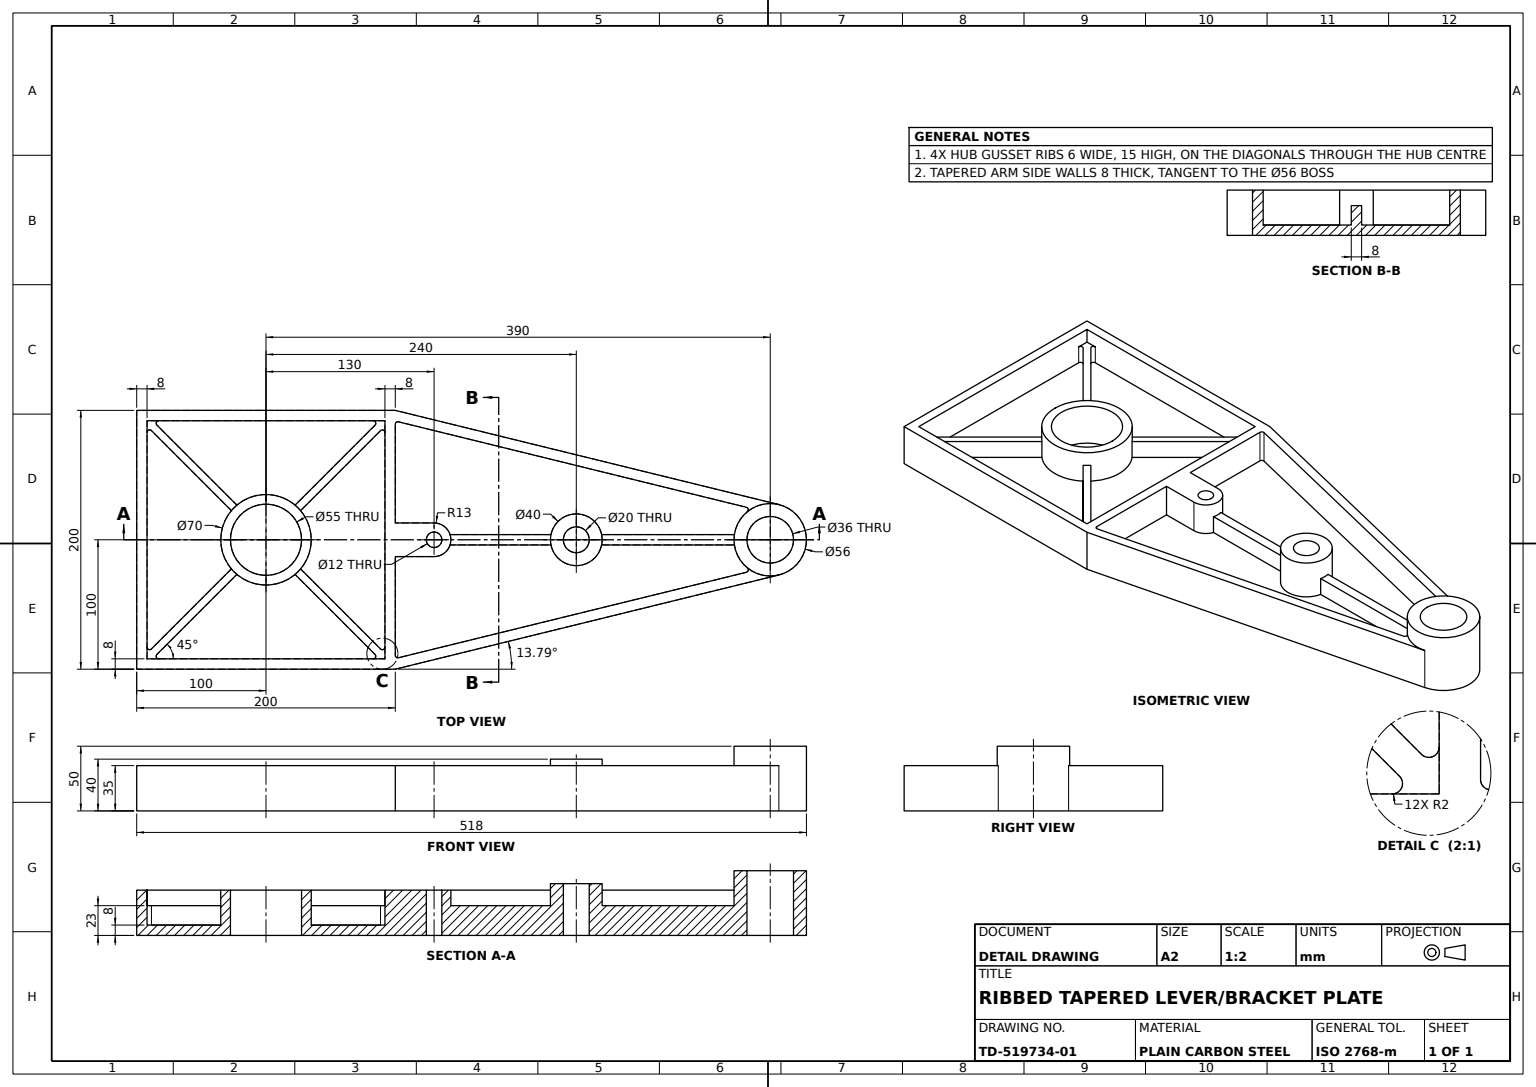
solid
v1 (92,8,-92)
v2 (91.816521,8,-92)
e1 v1 v2 LINE
v3 (92,35,-92)
e2 v3 v1 LINE
v4 (-92,35,-92)
e3 v3 v4 LINE
v5 (-92,8,-92)
e4 v4 v5 LINE
v6 (-91.816521,8,-92)
e5 v6 v5 LINE
v7 (-91.816521,23,-92)
e6 v6 v7 LINE
v8 (-82.913661,23,-92)
e7 v8 v7 LINE
v9 (-82.913661,8,-92)
e8 v8 v9 LINE
v10 (82.944203,8,-92)
e9 v10 v9 LINE
v11 (82.944203,23,-92)
e10 v10 v11 LINE
v12 (91.816521,23,-92)
e11 v12 v11 LINE
e12 v12 v2 LINE
face PLANE(AX(P(-92,35,-92),D(0,0,1),D(1,0,0))) [-e1 -e2 e3 e4 -e5 e6 -e7 e8 -e9 e10 -e11 e12]
v13 (-4,23,-220.404082)
v14 (-4,23,-142.369317)
e13 v13 v14 LINE
v15 (0,23,-143)
e14 v14 v15 CIRCLE(AX(P(0,23,-130),D(0,-1,0),D(0,0,-1)),13)
v16 (4,23,-142.369317)
e15 v15 v16 CIRCLE(AX(P(0,23,-130),D(0,-1,0),D(0,0,-1)),13)
v17 (4,23,-220.404082)
e16 v16 v17 LINE
v18 (0,23,-220)
e17 v17 v18 CIRCLE(AX(P(0,23,-240),D(0,-1,0),D(0,0,-1)),20)
e18 v18 v13 CIRCLE(AX(P(0,23,-240),D(0,-1,0),D(0,0,-1)),20)
face PLANE(AX(P(0,23,0),D(0,-1,0),D(0,0,-1))) rev [e13 e14 e15 e16 e17 e18]
v19 (-22.544627,23,26.771996)
v20 (-22.544627,8,26.771996)
e19 v19 v20 LINE
v21 (-84.358417,23,88.585786)
e20 v21 v19 LINE
v22 (-84.358417,8,88.585786)
e21 v21 v22 LINE
e22 v22 v20 LINE
face PLANE(AX(P(-89.794576,23,94.021945),D(-0.707106781,0,-0.707106781),D(-0.707106781,0,0.707106781))) rev [-e19 -e20 e21 e22]
v23 (92,23,91.816521)
v24 (92,8,91.816521)
e23 v23 v24 LINE
v25 (91.816521,23,92)
e24 v25 v23 LINE
v26 (91.816521,8,92)
e25 v26 v25 LINE
e26 v26 v24 LINE
face PLANE(AX(P(94.021945,23,89.794576),D(-0.707106781,0,-0.707106781),D(-0.707106781,0,0.707106781))) rev [-e23 -e24 -e25 e26]
v27 (25.14377,35,-371.458403)
v28 (25.14377,8,-371.458403)
e27 v27 v28 LINE
v29 (23.201406,35,-372.981725)
e28 v29 v27 CIRCLE(AX(P(23.201406,35,-370.981725),D(0,-1,0),D(0,0,1)),2)
v30 (23.201406,8,-372.981725)
e29 v29 v30 LINE
e30 v28 v30 CIRCLE(AX(P(23.201406,8,-370.981725),D(0,1,0),D(0,0,1)),2)
face CYL(AX(P(23.201406,8,-370.981725),D(0,-1,0),D(0,0,-1)),2) rev [-e27 -e28 e29 -e30]
v31 (-89.212448,35,-100)
v32 (-91.154812,35,-102.476677)
e31 v31 v32 CIRCLE(AX(P(-89.212448,35,-102),D(0,-1,0),D(0,0,1)),2)
v33 (-25.14377,35,-371.458403)
e32 v33 v32 LINE
v34 (-23.201406,35,-372.981725)
e33 v33 v34 CIRCLE(AX(P(-23.201406,35,-370.981725),D(0,-1,0),D(0,0,1)),2)
v35 (-21.654645,35,-372.24961)
e34 v34 v35 CIRCLE(AX(P(-23.201406,35,-370.981725),D(0,-1,0),D(0,0,1)),2)
v36 (-27.193099,35,-396.673482)
e35 v35 v36 CIRCLE(AX(P(0,35,-390),D(0,-1,0),D(0,0,1)),28)
v37 (-100,35,-100)
e36 v36 v37 LINE
v38 (-100,35,100)
e37 v37 v38 LINE
v39 (100,35,100)
e38 v38 v39 LINE
v40 (100,35,-100)
e39 v39 v40 LINE
v41 (27.193099,35,-396.673482)
e40 v40 v41 LINE
v42 (21.654645,35,-372.24961)
e41 v41 v42 CIRCLE(AX(P(0,35,-390),D(0,-1,0),D(0,0,1)),28)
e42 v42 v29 CIRCLE(AX(P(23.201406,35,-370.981725),D(0,-1,0),D(0,0,1)),2)
v43 (91.154812,35,-102.476677)
e43 v43 v27 LINE
v44 (89.212448,35,-100)
e44 v43 v44 CIRCLE(AX(P(89.212448,35,-102),D(0,-1,0),D(0,0,1)),2)
v45 (13,35,-100)
e45 v44 v45 LINE
v46 (13,35,-130)
e46 v45 v46 LINE
v47 (0,35,-143)
e47 v46 v47 CIRCLE(AX(P(0,35,-130),D(0,1,0),D(0,0,1)),13)
v48 (-13,35,-130)
e48 v47 v48 CIRCLE(AX(P(0,35,-130),D(0,1,0),D(0,0,1)),13)
v49 (-13,35,-100)
e49 v48 v49 LINE
e50 v49 v31 LINE
v50 (0,35,-136)
v51 (0,35,-124)
e51 v50 v51 CIRCLE(AX(P(0,35,-130),D(0,1,0),D(0,0,1)),6)
e52 v51 v50 CIRCLE(AX(P(0,35,-130),D(0,1,0),D(0,0,1)),6)
v52 (92,35,92)
e53 v52 v3 LINE
v53 (-92,35,92)
e54 v53 v52 LINE
e55 v4 v53 LINE
face PLANE(AX(P(0,35,0),D(0,1,0),D(0,0,1))) [e31 -e32 e33 e34 e35 e36 e37 e38 e39 e40 e41 e42 e28 -e43 e44 e45 e46 e47 e48 e49 e50] [-e51 -e52] [-e53 -e54 -e55 -e3]
v54 (-26.785954,23,22.528042)
v55 (-88.585786,23,84.327874)
e56 v54 v55 LINE
v56 (-26.785954,8,22.528042)
e57 v54 v56 LINE
v57 (-88.585786,8,84.327874)
e58 v56 v57 LINE
e59 v57 v55 LINE
face PLANE(AX(P(-94.037217,23,89.779305),D(0.707106781,0,0.707106781),D(0.707106781,0,-0.707106781))) rev [-e56 e57 e58 e59]
v58 (-21.654645,8,-372.24961)
v59 (-23.201406,8,-372.981725)
e60 v58 v59 CIRCLE(AX(P(-23.201406,8,-370.981725),D(0,1,0),D(0,0,1)),2)
e61 v35 v58 LINE
e62 v34 v59 LINE
face CYL(AX(P(-23.201406,8,-370.981725),D(0,-1,0),D(0,0,-1)),2) rev [-e60 -e61 -e34 e62]
v60 (0,50,-372)
v61 (0,0,-372)
e63 v60 v61 LINE
v62 (0,0,-408)
e64 v61 v62 CIRCLE(AX(P(0,0,-390),D(0,-1,0),D(0,0,-1)),18)
v63 (0,50,-408)
e65 v63 v62 LINE
e66 v60 v63 CIRCLE(AX(P(0,50,-390),D(0,-1,0),D(0,0,-1)),18)
face CYL(AX(P(0,50,-390),D(0,-1,0),D(0,0,-1)),18) rev [e63 e64 -e65 -e66]
v64 (-4,23,-362.287187)
v65 (-4,23,-259.595918)
e67 v64 v65 LINE
v66 (-4,8,-362.287187)
e68 v64 v66 LINE
v67 (-4,8,-259.595918)
e69 v66 v67 LINE
e70 v67 v65 LINE
face PLANE(AX(P(-4,23,-100.849632),D(1,0,0),D(0,0,-1))) rev [-e67 e68 e69 e70]
v68 (-13,8,-130)
v69 (-13,8,-100)
e71 v68 v69 LINE
e72 v49 v69 LINE
e73 v48 v68 LINE
face PLANE(AX(P(-13,85.249378,-130),D(1,0,0),D(0,0,-1))) rev [e71 -e72 -e49 e73]
e74 v47 v15 LINE
v70 (-4,8,-142.369317)
e75 v70 v14 LINE
e76 v70 v68 CIRCLE(AX(P(0,8,-130),D(0,1,0),D(0,0,1)),13)
face CYL(AX(P(0,85.249378,-130),D(0,-1,0),D(0,0,-1)),13) [-e48 e74 -e14 -e75 e76 -e73]
v71 (13,8,-130)
v72 (4,8,-142.369317)
e77 v71 v72 CIRCLE(AX(P(0,8,-130),D(0,1,0),D(0,0,1)),13)
e78 v16 v72 LINE
e79 v46 v71 LINE
face CYL(AX(P(0,85.249378,-130),D(0,-1,0),D(0,0,-1)),13) [e77 -e78 -e15 -e74 -e47 e79]
v73 (-89.212448,8,-100)
e80 v69 v73 LINE
e81 v73 v31 LINE
face PLANE(AX(P(-100,35,-100),D(0,0,1),D(1,0,0))) rev [e72 e80 e81 -e50]
v74 (-92,23,-91.816521)
v75 (-92,8,-91.816521)
e82 v74 v75 LINE
e83 v7 v74 LINE
e84 v6 v75 LINE
face PLANE(AX(P(-94.021945,23,-89.794576),D(0.707106781,0,0.707106781),D(0.707106781,0,-0.707106781))) rev [-e82 -e83 -e6 e84]
v76 (92,23,82.944203)
v77 (90,23,84.944203)
e85 v76 v77 CIRCLE(AX(P(90,23,82.944203),D(0,-1,0),D(0,0,1)),2)
v78 (88.585786,23,84.358417)
e86 v77 v78 CIRCLE(AX(P(90,23,82.944203),D(0,-1,0),D(0,0,1)),2)
v79 (26.771996,23,22.544627)
e87 v78 v79 LINE
v80 (22.528042,23,26.785954)
e88 v80 v79 CIRCLE(AX(P(0,23,0),D(0,1,0),D(0,0,1)),35)
v81 (84.327874,23,88.585786)
e89 v80 v81 LINE
v82 (82.913661,23,92)
e90 v81 v82 CIRCLE(AX(P(82.913661,23,90),D(0,-1,0),D(0,0,1)),2)
e91 v82 v25 LINE
e92 v23 v76 LINE
face PLANE(AX(P(0,23,0),D(0,1,0),D(0,0,1))) [e85 e86 e87 -e88 e89 e90 e91 e24 e92]
v83 (-88.585786,8,-84.358417)
v84 (-92,8,-82.944203)
e93 v83 v84 CIRCLE(AX(P(-90,8,-82.944203),D(0,1,0),D(0,0,1)),2)
v85 (-88.585786,23,-84.358417)
e94 v85 v83 LINE
v86 (-92,23,-82.944203)
e95 v86 v85 CIRCLE(AX(P(-90,23,-82.944203),D(0,-1,0),D(0,0,1)),2)
e96 v84 v86 LINE
face CYL(AX(P(-90,35,-82.944203),D(0,1,0),D(0,0,1)),2) rev [-e93 -e94 -e95 -e96]
v87 (21.654645,8,-372.24961)
e97 v30 v87 CIRCLE(AX(P(23.201406,8,-370.981725),D(0,1,0),D(0,0,1)),2)
e98 v87 v42 LINE
face CYL(AX(P(23.201406,8,-370.981725),D(0,-1,0),D(0,0,-1)),2) rev [-e97 -e29 -e42 -e98]
v88 (-92,8,91.816521)
v89 (-92,23,91.816521)
e99 v88 v89 LINE
v90 (-91.816521,8,92)
e100 v88 v90 LINE
v91 (-91.816521,23,92)
e101 v91 v90 LINE
e102 v89 v91 LINE
face PLANE(AX(P(-89.794576,23,94.021945),D(0.707106781,0,-0.707106781),D(-0.707106781,0,-0.707106781))) rev [-e99 e100 -e101 -e102]
v92 (-25.14377,8,-371.458403)
e103 v92 v33 LINE
e104 v59 v92 CIRCLE(AX(P(-23.201406,8,-370.981725),D(0,1,0),D(0,0,1)),2)
face CYL(AX(P(-23.201406,8,-370.981725),D(0,-1,0),D(0,0,-1)),2) rev [-e33 -e103 -e104 -e62]
v93 (82.913661,8,92)
v94 (84.327874,8,88.585786)
e105 v93 v94 CIRCLE(AX(P(82.913661,8,90),D(0,1,0),D(0,0,1)),2)
e106 v82 v93 LINE
e107 v94 v81 LINE
face CYL(AX(P(82.913661,35,90),D(0,-1,0),D(0,0,-1)),2) rev [-e105 -e106 -e90 -e107]
v95 (-4,8,-220.404082)
e108 v95 v70 LINE
e109 v13 v95 LINE
face PLANE(AX(P(-4,23,-100.849632),D(1,0,0),D(0,0,-1))) rev [e108 e75 -e13 e109]
v96 (-100,0,100)
e110 v38 v96 LINE
v97 (100,0,100)
e111 v96 v97 LINE
e112 v39 v97 LINE
face PLANE(AX(P(-100,8,100),D(0,0,-1),D(-1,0,0))) rev [-e38 e110 e111 -e112]
v98 (-82.944203,23,92)
e113 v98 v21 CIRCLE(AX(P(-82.944203,23,90),D(0,-1,0),D(0,0,1)),2)
e114 v54 v19 CIRCLE(AX(P(0,23,0),D(0,1,0),D(0,0,1)),35)
v99 (-92,23,82.913661)
e115 v55 v99 CIRCLE(AX(P(-90,23,82.913661),D(0,-1,0),D(0,0,1)),2)
e116 v99 v89 LINE
e117 v91 v98 LINE
face PLANE(AX(P(0,23,0),D(0,1,0),D(0,0,1))) [e113 e20 -e114 e56 e115 e116 e102 e117]
v100 (-91.154812,8,-102.476677)
e118 v32 v100 LINE
e119 v92 v100 LINE
face PLANE(AX(P(-89.799329,417.460455,-108),D(0.971182107,0,0.238338657),D(0.238338657,0,-0.971182107))) [e103 e32 e118 -e119]
e120 v74 v86 LINE
e121 v5 v75 LINE
v101 (-92,8,92)
e122 v53 v101 LINE
e123 v88 v101 LINE
v102 (-92,8,82.913661)
e124 v99 v102 LINE
e125 v84 v102 LINE
face PLANE(AX(P(-92,35,92),D(1,0,0),D(0,0,-1))) [e96 -e120 e82 -e121 -e4 e55 e122 -e123 e99 -e116 e124 -e125]
v103 (0,40,-230)
v104 (0,0,-230)
e126 v103 v104 LINE
v105 (0,0,-250)
e127 v104 v105 CIRCLE(AX(P(0,0,-240),D(0,-1,0),D(0,0,-1)),10)
v106 (0,40,-250)
e128 v106 v105 LINE
e129 v106 v103 CIRCLE(AX(P(0,40,-240),D(0,1,0),D(0,0,1)),10)
face CYL(AX(P(0,50,-240),D(0,-1,0),D(0,0,-1)),10) rev [e126 e127 -e128 e129]
v107 (-84.327874,8,-88.585786)
e130 v9 v107 CIRCLE(AX(P(-82.913661,8,-90),D(0,1,0),D(0,0,1)),2)
v108 (-22.528042,8,-26.785954)
e131 v108 v107 LINE
v109 (0,8,-35)
e132 v109 v108 CIRCLE(AX(P(0,8,0),D(0,1,0),D(0,0,1)),35)
v110 (22.544627,8,-26.771996)
e133 v110 v109 CIRCLE(AX(P(0,8,0),D(0,1,0),D(0,0,1)),35)
v111 (84.358417,8,-88.585786)
e134 v111 v110 LINE
e135 v111 v10 CIRCLE(AX(P(82.944203,8,-90),D(0,1,0),D(0,0,1)),2)
face PLANE(AX(P(0,8,-390),D(0,1,0),D(0,0,1))) [e130 -e131 -e132 -e133 -e134 e135 e9]
v112 (-84.327874,23,-88.585786)
e136 v107 v112 LINE
e137 v112 v8 CIRCLE(AX(P(-82.913661,23,-90),D(0,-1,0),D(0,0,1)),2)
face CYL(AX(P(-82.913661,35,-90),D(0,-1,0),D(0,0,-1)),2) rev [-e136 -e130 -e8 -e137]
v113 (88.585786,8,84.358417)
e138 v78 v113 LINE
v114 (90,8,84.944203)
e139 v114 v77 LINE
e140 v113 v114 CIRCLE(AX(P(90,8,82.944203),D(0,1,0),D(0,0,1)),2)
face CYL(AX(P(90,35,82.944203),D(0,1,0),D(0,0,1)),2) rev [-e138 -e86 -e139 -e140]
v115 (0,0,-136)
e141 v50 v115 LINE
v116 (0,0,-124)
e142 v115 v116 CIRCLE(AX(P(0,0,-130),D(0,-1,0),D(0,0,-1)),6)
e143 v51 v116 LINE
face CYL(AX(P(0,50,-130),D(0,-1,0),D(0,0,-1)),6) rev [e52 e141 e142 -e143]
v117 (-82.944203,8,92)
e144 v22 v117 CIRCLE(AX(P(-82.944203,8,90),D(0,1,0),D(0,0,1)),2)
e145 v117 v93 LINE
v118 (22.528042,8,26.785954)
e146 v118 v94 LINE
v119 (0,8,35)
e147 v119 v118 CIRCLE(AX(P(0,8,0),D(0,1,0),D(0,0,1)),35)
e148 v20 v119 CIRCLE(AX(P(0,8,0),D(0,1,0),D(0,0,1)),35)
face PLANE(AX(P(0,8,-390),D(0,1,0),D(0,0,1))) [e144 e145 e105 -e146 -e147 -e148 -e22]
v120 (0,23,-260)
e149 v65 v120 CIRCLE(AX(P(0,23,-240),D(0,-1,0),D(0,0,-1)),20)
v121 (4,23,-259.595918)
e150 v120 v121 CIRCLE(AX(P(0,23,-240),D(0,-1,0),D(0,0,-1)),20)
v122 (4,23,-362.287187)
e151 v121 v122 LINE
v123 (0,23,-362)
e152 v122 v123 CIRCLE(AX(P(0,23,-390),D(0,-1,0),D(0,0,-1)),28)
e153 v123 v64 CIRCLE(AX(P(0,23,-390),D(0,-1,0),D(0,0,-1)),28)
face PLANE(AX(P(0,23,0),D(0,-1,0),D(0,0,-1))) rev [e67 e149 e150 e151 e152 e153]
v124 (-26.771996,23,-22.544627)
e154 v85 v124 LINE
v125 (-22.528042,23,-26.785954)
e155 v125 v124 CIRCLE(AX(P(0,23,0),D(0,1,0),D(0,0,1)),35)
e156 v125 v112 LINE
face PLANE(AX(P(0,23,0),D(0,1,0),D(0,0,1))) [e7 e83 e120 e95 e154 -e155 e156 e137]
v126 (26.771996,8,22.544627)
e157 v113 v126 LINE
v127 (92,8,82.944203)
e158 v114 v127 CIRCLE(AX(P(90,8,82.944203),D(0,1,0),D(0,0,1)),2)
v128 (92,8,-82.913661)
e159 v127 v128 LINE
v129 (90,8,-84.913661)
e160 v128 v129 CIRCLE(AX(P(90,8,-82.913661),D(0,1,0),D(0,0,1)),2)
v130 (88.585786,8,-84.327874)
e161 v129 v130 CIRCLE(AX(P(90,8,-82.913661),D(0,1,0),D(0,0,1)),2)
v131 (26.785954,8,-22.528042)
e162 v131 v130 LINE
e163 v126 v131 CIRCLE(AX(P(0,8,0),D(0,1,0),D(0,0,1)),35)
face PLANE(AX(P(0,8,-390),D(0,1,0),D(0,0,1))) [-e157 e140 e158 e159 e160 e161 -e162 -e163]
v132 (84.358417,23,-88.585786)
e164 v11 v132 CIRCLE(AX(P(82.944203,23,-90),D(0,-1,0),D(0,0,1)),2)
e165 v132 v111 LINE
face CYL(AX(P(82.944203,35,-90),D(0,1,0),D(0,0,1)),2) rev [-e164 -e10 -e135 -e165]
e166 v103 v106 CIRCLE(AX(P(0,40,-240),D(0,1,0),D(0,0,1)),10)
e167 v105 v104 CIRCLE(AX(P(0,0,-240),D(0,-1,0),D(0,0,-1)),10)
face CYL(AX(P(0,50,-240),D(0,-1,0),D(0,0,-1)),10) rev [e166 e128 e167 -e126]
v133 (0,50,-362)
e168 v133 v123 LINE
v134 (0,50,-418)
e169 v134 v133 CIRCLE(AX(P(0,50,-390),D(0,1,0),D(0,0,1)),28)
v135 (0,0,-418)
e170 v134 v135 LINE
v136 (-27.193099,0,-396.673482)
e171 v135 v136 CIRCLE(AX(P(0,0,-390),D(0,1,0),D(0,0,1)),28)
e172 v36 v136 LINE
e173 v58 v66 CIRCLE(AX(P(0,8,-390),D(0,1,0),D(0,0,1)),28)
face CYL(AX(P(0,8,-390),D(0,-1,0),D(0,0,-1)),28) [-e153 -e168 -e169 e170 e171 -e172 -e35 e61 e173 -e68]
e174 v127 v76 LINE
face CYL(AX(P(90,35,82.944203),D(0,1,0),D(0,0,1)),2) rev [-e158 e139 -e85 -e174]
v137 (22.544627,23,-26.771996)
e175 v137 v110 LINE
v138 (0,35,-35)
e176 v138 v109 LINE
v139 (0,35,35)
e177 v139 v138 CIRCLE(AX(P(0,35,0),D(0,1,0),D(0,0,1)),35)
e178 v139 v119 LINE
e179 v80 v118 LINE
e180 v79 v126 LINE
v140 (26.785954,23,-22.528042)
e181 v140 v131 LINE
e182 v140 v137 CIRCLE(AX(P(0,23,0),D(0,1,0),D(0,0,1)),35)
face CYL(AX(P(0,35,0),D(0,-1,0),D(0,0,-1)),35) [e175 e133 -e176 -e177 e178 e147 -e179 e88 e180 e163 -e181 e182]
v141 (92,8,-91.816521)
e183 v141 v1 LINE
e184 v141 v2 LINE
face PLANE(AX(P(0,8,-390),D(0,1,0),D(0,0,1))) [e183 e1 -e184]
v142 (92,8,92)
e185 v26 v142 LINE
e186 v142 v24 LINE
face PLANE(AX(P(0,8,-390),D(0,1,0),D(0,0,1))) [e185 e186 -e26]
e187 v116 v115 CIRCLE(AX(P(0,0,-130),D(0,-1,0),D(0,0,-1)),6)
face CYL(AX(P(0,50,-130),D(0,-1,0),D(0,0,-1)),6) rev [-e141 e51 e143 e187]
v143 (0,0,27.5)
v144 (0,0,-27.5)
e188 v143 v144 CIRCLE(AX(P(0,0,0),D(0,-1,0),D(0,0,-1)),27.5)
v145 (0,35,-27.5)
e189 v145 v144 LINE
v146 (0,35,27.5)
e190 v145 v146 CIRCLE(AX(P(0,35,0),D(0,1,0),D(0,0,1)),27.5)
e191 v146 v143 LINE
face CYL(AX(P(0,50,0),D(0,-1,0),D(0,0,-1)),27.5) rev [e188 -e189 e190 e191]
v147 (-100,0,-100)
e192 v37 v147 LINE
e193 v147 v96 LINE
face PLANE(AX(P(-100,8,100),D(1,0,0),D(0,0,-1))) rev [-e110 -e37 e192 e193]
face PLANE(AX(P(94.021945,23,89.794576),D(-0.707106781,0,0.707106781),D(0.707106781,0,0.707106781))) rev [e138 e157 -e180 -e87]
e194 v144 v143 CIRCLE(AX(P(0,0,0),D(0,-1,0),D(0,0,-1)),27.5)
e195 v146 v145 CIRCLE(AX(P(0,35,0),D(0,1,0),D(0,0,1)),27.5)
face CYL(AX(P(0,50,0),D(0,-1,0),D(0,0,-1)),27.5) rev [e194 -e191 e195 e189]
v148 (100,0,-100)
e196 v97 v148 LINE
e197 v40 v148 LINE
face PLANE(AX(P(100,8,100),D(-1,0,0),D(0,0,1))) rev [-e39 e112 e196 -e197]
v149 (91.154812,8,-102.476677)
e198 v149 v28 LINE
e199 v149 v43 LINE
face PLANE(AX(P(19.423642,417.460455,-394.766773),D(-0.971182107,0,0.238338657),D(0.238338657,0,0.971182107))) [e27 -e198 e199 e43]
v150 (13,8,-100)
e200 v45 v150 LINE
e201 v150 v71 LINE
face PLANE(AX(P(13,85.249378,-130),D(-1,0,0),D(0,0,1))) rev [-e79 -e46 e200 e201]
e202 v102 v57 CIRCLE(AX(P(-90,8,82.913661),D(0,1,0),D(0,0,1)),2)
face CYL(AX(P(-90,35,82.913661),D(0,-1,0),D(0,0,-1)),2) rev [-e115 -e59 -e202 -e124]
e203 v117 v98 LINE
face CYL(AX(P(-82.944203,35,90),D(0,1,0),D(0,0,1)),2) rev [-e203 -e144 -e21 -e113]
e204 v136 v147 LINE
face PLANE(AX(P(-100,8,-100),D(0.971182107,0,0.238338657),D(0.238338657,0,-0.971182107))) rev [e204 -e192 -e36 e172]
v151 (89.212448,8,-100)
e205 v151 v150 LINE
e206 v151 v149 CIRCLE(AX(P(89.212448,8,-102),D(0,1,0),D(0,0,1)),2)
v152 (4,8,-362.287187)
e207 v152 v87 CIRCLE(AX(P(0,8,-390),D(0,1,0),D(0,0,1)),28)
v153 (4,8,-259.595918)
e208 v153 v152 LINE
v154 (4,8,-220.404082)
e209 v154 v153 CIRCLE(AX(P(0,8,-240),D(0,1,0),D(0,0,1)),20)
e210 v72 v154 LINE
face PLANE(AX(P(0,8,-390),D(0,1,0),D(0,0,1))) [-e201 -e205 e206 e198 e30 e97 -e207 -e208 -e209 -e210 -e77]
e211 v63 v60 CIRCLE(AX(P(0,50,-390),D(0,-1,0),D(0,0,-1)),18)
e212 v62 v61 CIRCLE(AX(P(0,0,-390),D(0,-1,0),D(0,0,-1)),18)
face CYL(AX(P(0,50,-390),D(0,-1,0),D(0,0,-1)),18) rev [-e63 -e211 e65 e212]
v155 (92,23,-91.816521)
e213 v155 v12 LINE
e214 v141 v155 LINE
face PLANE(AX(P(89.794576,23,-94.021945),D(-0.707106781,0,0.707106781),D(0.707106781,0,0.707106781))) rev [-e213 -e214 e184 -e12]
v156 (-26.771996,8,-22.544627)
e215 v124 v156 LINE
e216 v156 v56 CIRCLE(AX(P(0,8,0),D(0,1,0),D(0,0,1)),35)
e217 v138 v139 CIRCLE(AX(P(0,35,0),D(0,1,0),D(0,0,1)),35)
e218 v125 v108 LINE
face CYL(AX(P(0,35,0),D(0,-1,0),D(0,0,-1)),35) [e215 e216 -e57 e114 e19 e148 -e178 -e217 e176 e132 -e218 e155]
e219 v83 v156 LINE
face PLANE(AX(P(-94.021945,23,-89.794576),D(0.707106781,0,-0.707106781),D(-0.707106781,0,-0.707106781))) rev [-e154 e94 e219 -e215]
v157 (27.193099,0,-396.673482)
e220 v41 v157 LINE
e221 v157 v135 CIRCLE(AX(P(0,0,-390),D(0,1,0),D(0,0,1)),28)
e222 v133 v134 CIRCLE(AX(P(0,50,-390),D(0,1,0),D(0,0,1)),28)
e223 v152 v122 LINE
face CYL(AX(P(0,8,-390),D(0,-1,0),D(0,0,-1)),28) [e98 -e41 e220 e221 -e170 -e222 e168 -e152 -e223 e207]
e224 v44 v151 LINE
face PLANE(AX(P(-100,35,-100),D(0,0,1),D(1,0,0))) rev [e224 e205 -e200 -e45]
v158 (0,40,-260)
e225 v158 v120 LINE
v159 (0,40,-220)
e226 v159 v158 CIRCLE(AX(P(0,40,-240),D(0,1,0),D(0,0,1)),20)
e227 v159 v18 LINE
e228 v154 v17 LINE
e229 v121 v153 LINE
face CYL(AX(P(0,40,-240),D(0,-1,0),D(0,0,-1)),20) [-e225 -e226 e227 -e17 -e228 e209 -e229 -e150]
e230 v52 v142 LINE
e231 v101 v90 LINE
face PLANE(AX(P(-92,35,92),D(0,0,-1),D(-1,0,0))) [e230 -e185 e25 -e91 e106 -e145 e203 -e117 e101 -e231 -e122 e54]
e232 v67 v95 CIRCLE(AX(P(0,8,-240),D(0,1,0),D(0,0,1)),20)
e233 v158 v159 CIRCLE(AX(P(0,40,-240),D(0,1,0),D(0,0,1)),20)
face CYL(AX(P(0,40,-240),D(0,-1,0),D(0,0,-1)),20) [e232 -e109 -e18 -e227 -e233 e225 -e149 -e70]
face PLANE(AX(P(0,35,0),D(0,1,0),D(0,0,1))) [-e190 -e195] [e177 e217]
v160 (92,23,-82.913661)
e234 v160 v155 LINE
e235 v160 v128 LINE
face PLANE(AX(P(92,35,92),D(-1,0,0),D(0,0,1))) [e2 -e183 e214 -e234 e235 -e159 e174 -e92 e23 -e186 -e230 e53]
e236 v132 v137 LINE
face PLANE(AX(P(89.794576,23,-94.021945),D(0.707106781,0,0.707106781),D(0.707106781,0,-0.707106781))) rev [e134 -e175 -e236 e165]
face PLANE(AX(P(0,8,-390),D(0,1,0),D(0,0,1))) [-e100 e123 e231]
v161 (88.585786,23,-84.327874)
e237 v140 v161 LINE
v162 (90,23,-84.913661)
e238 v161 v162 CIRCLE(AX(P(90,23,-82.913661),D(0,-1,0),D(0,0,1)),2)
e239 v162 v160 CIRCLE(AX(P(90,23,-82.913661),D(0,-1,0),D(0,0,1)),2)
face PLANE(AX(P(0,23,0),D(0,1,0),D(0,0,1))) [-e182 e237 e238 e239 e234 e213 e11 e164 e236]
face PLANE(AX(P(-89.779305,23,-94.037217),D(-0.707106781,0,0.707106781),D(0.707106781,0,0.707106781))) rev [e131 e136 -e156 e218]
face PLANE(AX(P(89.779305,23,94.037217),D(0.707106781,0,-0.707106781),D(-0.707106781,0,-0.707106781))) rev [e146 e107 -e89 e179]
e240 v130 v161 LINE
face PLANE(AX(P(94.037217,23,-89.779305),D(-0.707106781,0,-0.707106781),D(-0.707106781,0,0.707106781))) rev [e162 e240 -e237 e181]
e241 v148 v157 LINE
face PLANE(AX(P(0,0,-390),D(0,1,0),D(0,0,1))) rev [-e64 -e212] [-e127 -e167] [-e142 -e187] [-e221 -e241 -e196 -e111 -e193 -e204 -e171] [-e194 -e188]
face PLANE(AX(P(0,40,-240),D(0,1,0),D(0,0,1))) [-e129 -e166] [e226 e233]
e242 v100 v73 CIRCLE(AX(P(-89.212448,8,-102),D(0,1,0),D(0,0,1)),2)
face PLANE(AX(P(0,8,-390),D(0,1,0),D(0,0,1))) [e242 -e80 -e71 -e76 -e108 -e232 -e69 -e173 e60 e104 e119]
face PLANE(AX(P(4,23,-100.849632),D(-1,0,0),D(0,0,1))) rev [e228 -e16 e78 e210]
face CYL(AX(P(89.212448,35,-102),D(0,-1,0),D(0,0,-1)),2) rev [-e199 -e206 -e224 -e44]
e243 v162 v129 LINE
face CYL(AX(P(90,35,-82.913661),D(0,-1,0),D(0,0,-1)),2) rev [-e235 -e239 e243 -e160]
face PLANE(AX(P(0,50,-390),D(0,1,0),D(0,0,1))) [e211 e66] [e222 e169]
face CYL(AX(P(-89.212448,417.460455,-102),D(0,-1,0),D(0,0,-1)),2) rev [-e31 -e81 -e242 -e118]
face PLANE(AX(P(100,8,-100),D(-0.971182107,0,0.238338657),D(0.238338657,0,0.971182107))) rev [-e40 e197 e241 -e220]
face PLANE(AX(P(0,8,-390),D(0,1,0),D(0,0,1))) [e5 e121 -e84]
face PLANE(AX(P(4,23,-100.849632),D(-1,0,0),D(0,0,1))) rev [e208 e223 -e151 e229]
face CYL(AX(P(90,35,-82.913661),D(0,-1,0),D(0,0,-1)),2) rev [-e243 -e238 -e240 -e161]
face PLANE(AX(P(0,8,-390),D(0,1,0),D(0,0,1))) [e125 e202 -e58 -e216 -e219 e93]
